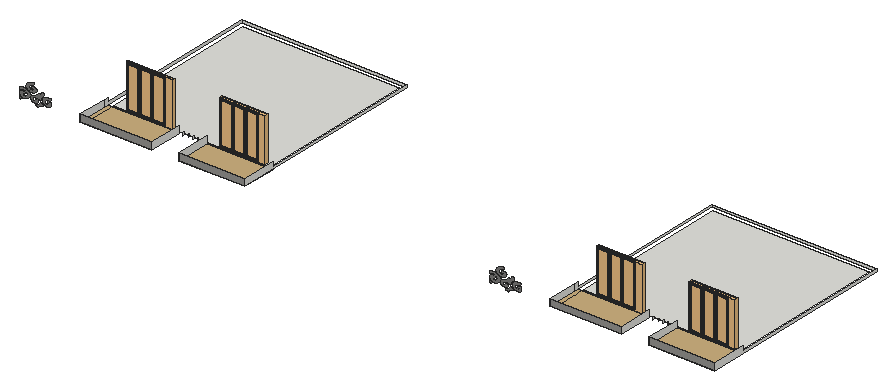
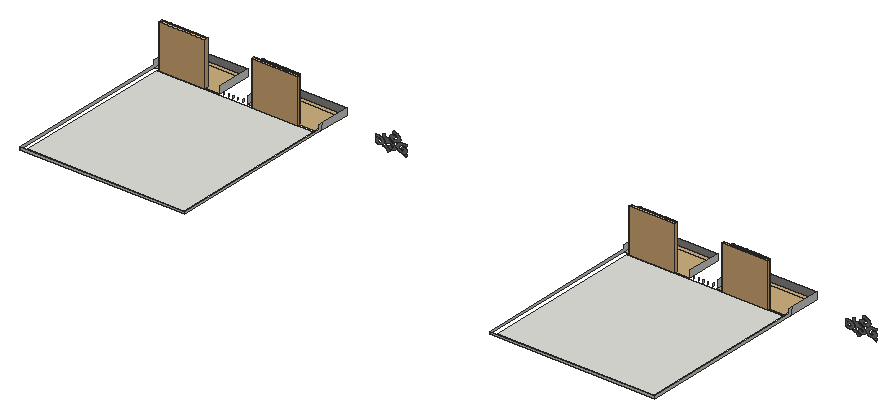
# SketchUp Ruby script. Lengths in inches.
U = 1.inch
M = Sketchup.active_model
def pt(a) = Geom::Point3d.new(a.map { |v| v * U })
def face(e, loops, mat)
  f = e.add_face(loops[0].map { |a| pt(a) })
  loops[1..].each { |l| e.add_face(l.map { |a| pt(a) }).erase! }
  f.material = f.back_material = mat if mat
  f
end
# faces: each face lists its corners as indices into pts; further lists are holes
def faces(e, pts, list, mat = nil) = list.each { |f| face(e, (f[0].is_a?(Array) ? f : [f]).map { |l| l.map { |i| pts[i] } }, mat) }
# xy, xz, yz: faces in a plane at the given z, y or x. An outline is a flat list of corners, or four numbers for a rectangle; further outlines are holes
def ring(l) = l.size == 4 ? [[l[0], l[1]], [l[2], l[1]], [l[2], l[3]], [l[0], l[3]]] : l.each_slice(2).to_a
def flat(e, list, mat, &to3) = list.each { |f| face(e, (f[0].is_a?(Array) ? f : [f]).map { |l| ring(l).map { |u, v| to3.(u, v) } }, mat) }
def xy(e, z, list, mat = nil) = flat(e, list, mat) { |x, y| [x, y, z] }
def xz(e, y, list, mat = nil) = flat(e, list, mat) { |x, z| [x, y, z] }
def yz(e, x, list, mat = nil) = flat(e, list, mat) { |y, z| [x, y, z] }
def lines(e, pts, list) = list.each { |a, b| e.add_line(pt(pts[a]), pt(pts[b])) }
# prism: a flat outline (further loops are holes) pulled along v
def prism(e, loops, v, mat = nil)
  f = face(e, loops, mat); d = Geom::Vector3d.new(v.map { |x| x * U })
  f.pushpull(f.normal.samedirection?(d) ? d.length : -d.length)
end
def box(e, o, s, mat = nil) = prism(e, [[o, [o[0] + s[0], o[1], o[2]], [o[0] + s[0], o[1] + s[1], o[2]], [o[0], o[1] + s[1], o[2]]]], [0, 0, s[2]], mat)
def at(x, y, z, deg = 0) = Geom::Transformation.translation(pt([x, y, z])) * Geom::Transformation.rotation(ORIGIN, Z_AXIS, deg.degrees)
def axes(o, x, y, z) = Geom::Transformation.new([*x, 0, *y, 0, *z, 0, *pt(o).to_a, 1])
def part(name) = M.definitions.add(name)
# library, detail: a bought-in or finely detailed component or shape, given as its bounding box
def library(name, o, s) = part(name).tap { |d| box(d.entities, o, s) }
def detail(e, o, s) = box(e.add_group.entities, o, s)
def put(e, d, t, mat = nil) = e.add_instance(d, t).tap { |i| i.material = mat if mat }
def group(e, t, mat = nil) = e.add_group.tap { |g| g.transformation = t; g.material = mat if mat }.entities
root = M.entities
M.materials.add("Wine2").color = [0, 0, 0]
M.materials["Wine2"].alpha = 0
M.materials.add("[0043_SaddleBrown]4").color = [124, 123, 122]
M.materials.add("[0130_Gainsboro]").color = [39, 45, 50]
M.materials.add("[Granite Light Gray]").color = [149, 148, 144]
M.materials.add("[Wood Floor Light]").color = [204, 176, 127]
c1 = part("Framed glazing panel")
xy(c1.entities,0,[[0,-0.98,43.07,0],[0,0,43.07,1.4]],"[0130_Gainsboro]")
xy(c1.entities,0.3,[[0.3,-1.43,42.77,-0.98]],"[0130_Gainsboro]")
xy(c1.entities,2.95,[[2.95,-1.43,40.12,-0.63],[2.95,-0.63,40.12,0],[2.95,0,40.12,0.64],[2.95,0.64,40.12,1.4]],"[0130_Gainsboro]")
xy(c1.entities,3.54,[[3.54,-0.63,39.53,0],[3.54,0,39.53,0.64]],"[0130_Gainsboro]")
xy(c1.entities,111.8125,[[3.54,-0.63,39.53,0],[3.54,0,39.53,0.64]],"[0130_Gainsboro]")
xy(c1.entities,112.4,[[2.95,-1.43,40.12,-0.63],[2.95,-0.63,40.12,0],[2.95,0,40.12,0.64],[2.95,0.64,40.12,1.4]],"[0130_Gainsboro]")
xy(c1.entities,115.05,[[0.3,-1.43,42.77,-0.98]],"[0130_Gainsboro]")
xy(c1.entities,115.35,[[0,-0.98,43.07,0],[0,0,43.07,1.4]],"[0130_Gainsboro]")
xz(c1.entities,-1.43,[[[0.3,0.3,42.77,115.05],[2.95,2.95,40.12,112.4]]],"[0130_Gainsboro]")
xz(c1.entities,-0.98,[[[0,0,43.07,115.35],[0.3,0.3,42.77,115.05]]],"[0130_Gainsboro]")
xz(c1.entities,-0.63,[[[2.95,2.95,40.12,112.4],[3.54,3.54,39.53,111.8125]]],"[0130_Gainsboro]")
xz(c1.entities,0,[[3.54,3.54,39.53,111.8125]],"Wine2")
xz(c1.entities,0,[[[0,0,43.07,115.35],[2.95,2.95,40.12,112.4]],[[2.95,2.95,40.12,112.4],[3.54,3.54,39.53,111.8125]]],"[0130_Gainsboro]")
xz(c1.entities,0.64,[[[2.95,2.95,40.12,112.4],[3.54,3.54,39.53,111.8125]]],"[0130_Gainsboro]")
xz(c1.entities,1.4,[[[0,0,43.07,115.35],[2.95,2.95,40.12,112.4]]],"[0130_Gainsboro]")
yz(c1.entities,0,[[-0.98,0,0,115.35],[0,0,1.4,115.35]],"[0130_Gainsboro]")
yz(c1.entities,0.3,[[-1.43,0.3,-0.98,115.05]],"[0130_Gainsboro]")
yz(c1.entities,2.95,[[-1.43,2.95,-0.63,112.4],[-0.63,2.95,0,112.4],[0,2.95,0.64,112.4],[0.64,2.95,1.4,112.4]],"[0130_Gainsboro]")
yz(c1.entities,3.54,[[-0.63,3.54,0,111.8125],[0,3.54,0.64,111.8125]],"[0130_Gainsboro]")
yz(c1.entities,39.53,[[-0.63,3.54,0,111.8125],[0,3.54,0.64,111.8125]],"[0130_Gainsboro]")
yz(c1.entities,40.12,[[-1.43,2.95,-0.63,112.4],[-0.63,2.95,0,112.4],[0,2.95,0.64,112.4],[0.64,2.95,1.4,112.4]],"[0130_Gainsboro]")
yz(c1.entities,42.77,[[-1.43,0.3,-0.98,115.05]],"[0130_Gainsboro]")
yz(c1.entities,43.07,[[-0.98,0,0,115.35],[0,0,1.4,115.35]],"[0130_Gainsboro]")
c2 = part("Glazing assembly")
put(c2.entities,c1,axes([90.57,1.43,0],[1.05148,0,0],[0,1,0],[0,0,1]))
put(c2.entities,c1,axes([0,1.43,0],[1.05148,0,0],[0,1,0],[0,0,1]))
put(c2.entities,c1,axes([45.29,1.43,0],[1.05148,0,0],[0,1,0],[0,0,1]))
c3 = library("Curtains",[0,0,0],[121.73,8.19,117.22])
xy(root,514.875,[[602.01,651.03,703.26,657.03],[849.76,651.03,951.01,657.03],[1852.64,651.03,1953.89,657.03],[2100.38,651.03,2201.63,657.03]])
xy(root,520.4375,[[563.08,657.03,978.86,1085.17],[1813.71,657.03,2229.49,1085.17]])
xy(root,520.4375,[[551.76,559.875,742.44,570.83],[814.89,559.875,990.19,570.83],[1802.38,559.875,1993.07,570.83],[2065.52,559.875,2240.81,570.83],[551.76,570.83,563.08,651.03],
  [563.08,570.83,742.44,651.03],[814.89,570.83,978.86,651.03],[978.86,570.83,990.19,651.03],[1802.38,570.83,1813.71,651.03],[1813.71,570.83,1993.07,651.03],
  [2065.52,570.83,2229.49,651.03],[2229.49,570.83,2240.81,651.03]],"[Wood Floor Light]")
xz(root,559.875,[[551.76,520.4375,742.44,538.1875],[814.89,520.4375,990.19,538.1875],[1802.38,520.4375,1993.07,538.1875],[2065.52,520.4375,2240.81,538.1875]],"[Granite Light Gray]")
xz(root,589.17,[[416.88,494.52,416.4,494.86,415.89,495.2,415.37,495.53,414.83,495.84,414.27,496.14,413.69,496.43,413.09,496.71,412.48,496.97,411.86,497.21,411.22,497.45,410.56,497.67,409.89,497.87,411.46,498.36,412.96,498.91,414.39,499.53,415.75,500.21,417.03,500.95,418.22,501.74,419.3125,502.59,420.3,503.48,421.19,504.4,421.97,505.37,422.63,506.37,423.18,507.39,423.73,507,424.29,506.61,424.86,506.23,425.44,505.86,426.04,505.49,426.64,505.13,427.25,504.77,427.87,504.42,429.13,503.74,429.78,503.41,430.4375,503.08,428.78,502.8125,427.17,502.44,425.625,501.98,424.16,501.42,422.8,500.78,421.54,500.0625,420.4,499.27,419.4,498.42,418.54,497.5,417.83,496.54,417.27,495.54],[1667.5,494.52,1667.02,494.86,1666.52,495.2,1666,495.53,1665.45,495.84,1664.89,496.14,1664.31,496.43,1663.72,496.71,1663.11,496.97,1662.48,497.21,1661.84,497.45,1661.19,497.67,1660.52,497.87,1662.08,498.36,1663.58,498.91,1665.02,499.53,1666.38,500.21,1667.66,500.95,1668.84,501.74,1669.9375,502.59,1670.93,503.48,1671.82,504.4,1672.59,505.37,1673.26,506.37,1673.8,507.39,1674.35,507,1674.92,506.61,1675.49,506.23,1676.07,505.86,1676.66,505.49,1677.26,505.13,1677.87,504.77,1678.49,504.42,1679.12,504.08,1679.76,503.74,1680.41,503.41,1681.0625,503.08,1679.4,502.8125,1677.79,502.44,1676.25,501.98,1674.79,501.42,1673.42,500.78,1672.16,500.0625,1671.03,499.27,1670.03,498.42,1669.16,497.5,1668.45,496.54,1667.9,495.54],[368.68,499.68,368.68,504.25,369.1,503.96,369.54,503.69,369.99,503.43,370.46,503.18,370.96,502.95,371.46,502.73,371.99,502.52,372.52,502.32,373.64,501.98,374.21,501.83,374.8,501.7,374.42,501.42,374.01,501.16,373.57,500.91,373.1,500.68,372.61,500.48,372.09,500.29,371.56,500.13,371.01,499.99,370.4375,499.875,369.86,499.78,369.28,499.72],[1619.31,499.68,1619.31,504.25,1619.72,503.96,1620.16,503.69,1620.62,503.43,1621.09,503.18,1621.58,502.95,1622.09,502.73,1622.61,502.52,1623.15,502.32,1623.7,502.15,1624.26,501.98,1624.84,501.83,1625.42,501.7,1625.04,501.42,1624.63,501.16,1624.19,500.91,1623.72,500.68,1623.23,500.48,1622.72,500.29,1622.18,500.13,1621.63,499.99,1621.0625,499.875,1620.49,499.78,1619.9,499.72],[406.11,502.53,404.67,502.63,403.28,502.875,401.97,503.24,400.76,503.73,399.6875,504.32,398.77,505.01,398.04,505.77,397.5,506.59,397.17,507.46,397.0625,508.34,396.95,509.36,397.01,510.38,397.25,511.39,397.65,512.39,398.22,513.35,398.95,514.27,399.83,515.14,400.85,515.94,402,516.68,403.27,517.34,404.64,517.92,406.1,518.41,407.49,518.85,408.83,519.35,410.1,519.91,411.3,520.53,412.43,521.19,413.49,521.91,414.45,522.66,415.33,523.46,416.11,524.29,416.79,525.16,417.38,526.05,417.86,526.96,418.53,526.65,419.27,526.39,420.07,526.2,420.89,526.08,421.74,526.02,422.59,526.04,423.42,526.13,424.24,526.28,425,526.51,425.72,526.79,426.36,527.13,426.92,527.52,427.13,527.84,427.28,528.17,427.36,528.51,427.38,528.85,427.34,529.18,427.24,529.52,427.08,529.85,426.86,530.16,426.58,530.45,426.25,530.73,425.875,530.98,425.45,531.2,425.22,531.33,425.04,531.48,424.91,531.66,424.84,531.85,424.83,532.04,424.875,532.23,424.98,532.41,425.15,532.57,425.36,532.71,425.61,532.83,425.9,532.91,426.2,532.95,426.76,532.98,427.32,532.95,427.86,532.875,428.38,532.75,428.87,532.59,429.32,532.38,429.71,532.14,430.04,531.86,430.31,531.56,430.5,531.24,430.61,530.9,430.65,530.56,430.86,529.99,431.01,529.41,431.09,528.83,431.09,528.24,431.03,527.66,430.9,527.08,430.7,526.5,430.43,525.94,430.1,525.39,429.7,524.86,429.24,524.35,428.72,523.86,427.79,523,426.92,522.11,426.11,521.2,425.375,520.27,424.71,519.33,424.11,518.36,423.59,517.375,423.14,516.38,422.76,515.375,422.46,514.36,422.23,513.33,422.08,512.3,421.11,513.07,419.99,513.75,418.74,514.33,417.37,514.8125,415.91,515.18,414.39,515.42,412.83,515.55,411.25,515.54,409.6875,515.42,408.17,515.16,406.71,514.79,405.35,514.31,404.375,513.85,403.51,513.32,402.76,512.72,402.14,512.07,401.66,511.38,401.33,510.65,401.16,509.91,401.14,509.15,401.28,508.41,401.58,507.67,402.03,506.97,402.62,506.3125,403.16,506.0625,403.76,505.86,404.41,505.72,405.08,505.64,405.76,505.62,406.4375,505.66,407.1,505.77,407.73,505.93,408.31,506.16,408.83,506.43,409.28,506.74,409.64,507.1,409.52,507.35,409.4375,507.61,409.38,507.87,409.36,508.125,409.38,508.39,409.43,508.65,409.51,508.91,409.62,509.16,409.77,509.4,409.94,509.64,410.15,509.87,410.39,510.09,410.62,510.26,410.89,510.4,411.2,510.51,411.53,510.6,411.88,510.65,412.24,510.67,412.59,510.65,412.94,510.6,413.27,510.51,413.58,510.4,413.85,510.26,414.08,510.09,414.76,509.4,415.23,508.65,415.49,507.87,415.52,507.07,415.33,506.27,414.92,505.51,414.3125,504.8,413.51,504.17,412.55,503.63,411.45,503.2,410.24,502.89,408.97,502.71,407.55,502.55],
  [1656.73,502.53,1655.3,502.63,1653.91,502.875,1652.59,503.24,1651.39,503.73,1650.3125,504.32,1649.4,505.01,1648.66,505.77,1648.125,506.59,1647.8,507.46,1647.6875,508.34,1647.58,509.36,1647.64,510.38,1647.87,511.39,1648.28,512.39,1648.84,513.35,1649.57,514.27,1650.45,515.14,1651.47,515.94,1652.62,516.68,1653.89,517.34,1655.27,517.92,1656.73,518.41,1658.12,518.85,1659.45,519.35,1660.72,519.91,1661.93,520.53,1663.06,521.19,1664.11,521.91,1665.08,522.66,1665.95,523.46,1666.74,524.29,1667.42,525.16,1668,526.05,1668.48,526.96,1669.16,526.65,1669.9,526.39,1670.69,526.2,1671.52,526.08,1672.36,526.02,1673.21,526.04,1674.05,526.13,1674.86,526.28,1675.63,526.51,1676.34,526.79,1676.99,527.13,1677.55,527.52,1677.75,527.84,1677.9,528.17,1677.99,528.51,1678.01,528.85,1677.97,529.18,1677.87,529.52,1677.7,529.85,1677.48,530.16,1677.21,530.45,1676.875,530.73,1676.5,530.98,1676.08,531.2,1675.85,531.33,1675.66,531.48,1675.53,531.66,1675.46,531.85,1675.45,532.04,1675.5,532.23,1675.61,532.41,1675.77,532.57,1675.99,532.71,1676.24,532.83,1676.52,532.91,1676.83,532.95,1677.38,532.98,1677.94,532.95,1678.49,532.875,1679.01,532.75,1679.5,532.59,1679.94,532.38,1680.33,532.14,1680.67,531.86,1680.93,531.56,1681.12,531.24,1681.24,530.9,1681.27,530.56,1681.49,529.99,1681.63,529.41,1681.71,528.83,1681.72,528.24,1681.66,527.66,1681.52,527.08,1681.32,526.5,1681.06,525.94,1680.72,525.39,1680.33,524.86,1679.87,524.35,1679.35,523.86,1678.41,523,1677.54,522.11,1676.74,521.2,1676,520.27,1675.33,519.33,1674.74,518.36,1674.21,517.375,1673.76,516.38,1673.38,515.375,1673.08,514.36,1672.86,513.33,1672.7,512.3,1671.74,513.07,1670.62,513.75,1669.36,514.33,1667.99,514.8125,1666.54,515.18,1665.01,515.42,1663.45,515.55,1661.875,515.54,1660.3125,515.42,1658.79,515.16,1657.34,514.79,1655.97,514.31,1655,513.85,1654.13,513.32,1653.38,512.72,1652.76,512.07,1652.29,511.38,1651.96,510.65,1651.78,509.91,1651.77,509.15,1651.91,508.41,1652.2,507.67,1652.65,506.97,1653.24,506.3125,1653.79,506.0625,1654.39,505.86,1655.03,505.72,1655.7,505.64,1656.38,505.62,1657.0625,505.66,1657.72,505.77,1658.35,505.93,1658.93,506.16,1659.45,506.43,1659.9,506.74,1660.27,507.1,1660.15,507.35,1660.0625,507.61,1660.01,507.87,1659.99,508.125,1660,508.39,1660.05,508.65,1660.13,508.91,1660.25,509.16,1660.39,509.4,1660.57,509.64,1660.78,509.87,1661.01,510.09,1661.25,510.26,1661.52,510.4,1661.82,510.51,1662.16,510.6,1662.5,510.65,1662.86,510.67,1663.22,510.65,1663.57,510.6,1663.9,510.51,1664.2,510.4,1664.48,510.26,1664.71,510.09,1665.38,509.4,1665.85,508.65,1666.11,507.87,1666.15,507.07,1665.96,506.27,1665.55,505.51,1664.9375,504.8,1664.14,504.17,1663.17,503.63,1662.07,503.2,1660.87,502.89,1659.59,502.71,1658.17,502.55],[378.83,503.5,377.68,503.64,376.54,503.84,375.45,504.11,374.4,504.44,373.4,504.83,372.47,505.28,371.62,505.78,370.84,506.32,370.15,506.91,369.5625,507.54,369.07,508.2,368.68,508.88,368.68,515.77,369.21,516.54,369.99,517.23,370.98,517.81,372.13,518.25,373.41,518.54,374.76,518.66,376.12,518.61,377.4375,518.39,378.66,518.01,379.72,517.49,380.59,516.85,381.23,516.11,381.32,515.93,381.375,515.75,381.38,515.56,381.34,515.375,381.26,515.19,381.13,515.02,380.97,514.87,380.76,514.72,380.53,514.6,380.27,514.51,379.99,514.43,379.7,514.38,378.97,514.46,378.24,514.45,377.51,514.36,376.83,514.19,376.21,513.95,375.67,513.64,375.24,513.27,374.92,512.86,374.74,512.42,374.68,511.97,374.76,511.52,374.98,511.09,375.16,510.53,375.49,509.99,375.94,509.49,376.52,509.04,377.21,508.65,377.99,508.34,378.84,508.1,379.74,507.95,380.67,507.89,381.6,507.91,382.51,508.03,383.39,508.24,384.74,508.91,385.93,509.6875,386.93,510.5625,387.71,511.52,388.27,512.53,388.59,513.58,388.66,514.65,388.49,515.71,388.07,516.75,387.42,517.74,386.54,518.67,385.47,519.51,385.03,520.06,384.51,520.6,383.93,521.1,383.28,521.57,382.57,522.01,381.81,522.41,380.99,522.77,380.12,523.08,379.22,523.35,378.28,523.58,377.32,523.75,376.33,523.875,375.63,523.93,374.92,523.94,374.22,523.92,373.52,523.86,372.83,523.77,372.15,523.64,371.5,523.48,370.87,523.28,370.27,523.05,369.7,522.8,369.17,522.51,368.68,522.2,368.68,526.94,370.83,527.38,373.04,527.66,375.3,527.78,377.56,527.72,379.79,527.51,381.97,527.125,384.05,526.59,386.02,525.9,387.84,525.07,389.48,524.12,390.93,523.05,392.16,521.88,393.82,520.15,394.98,518.26,395.59,516.28,395.64,514.26,395.12,512.26,394.05,510.36,392.45,508.59,390.39,507.02,387.92,505.69,385.11,504.64,382.05,503.91],[1629.46,503.5,1628.3,503.64,1627.17,503.84,1626.07,504.11,1625.02,504.44,1624.03,504.83,1623.1,505.28,1622.24,505.78,1621.47,506.32,1620.78,506.91,1620.1875,507.54,1619.7,508.2,1619.31,508.88,1619.31,515.77,1619.84,516.54,1620.61,517.23,1621.6,517.81,1622.76,518.25,1624.04,518.54,1625.39,518.66,1626.75,518.61,1628.0625,518.39,1629.28,518.01,1630.35,517.49,1631.22,516.85,1631.86,516.11,1631.95,515.93,1632,515.75,1632,515.56,1631.97,515.375,1631.88,515.19,1631.76,515.02,1631.59,514.87,1631.39,514.72,1631.16,514.6,1630.9,514.51,1630.62,514.43,1630.32,514.38,1629.6,514.46,1628.86,514.45,1628.14,514.36,1627.46,514.19,1626.84,513.95,1626.3,513.64,1625.87,513.27,1625.55,512.86,1625.36,512.42,1625.31,511.97,1625.39,511.52,1625.6,511.09,1625.79,510.53,1626.11,509.99,1626.57,509.49,1627.15,509.04,1627.84,508.65,1628.62,508.34,1629.47,508.1,1630.37,507.95,1631.29,507.89,1632.23,507.91,1633.14,508.03,1634.01,508.24,1635.37,508.91,1636.56,509.6875,1637.55,510.5625,1638.34,511.52,1638.89,512.53,1639.21,513.58,1639.28,514.65,1639.11,515.71,1638.69,516.75,1638.04,517.74,1637.17,518.67,1636.09,519.51,1635.65,520.06,1635.14,520.6,1634.56,521.1,1633.91,521.57,1633.2,522.01,1632.43,522.41,1631.61,522.77,1630.75,523.08,1629.84,523.35,1628.91,523.58,1627.94,523.75,1626.96,523.875,1626.25,523.93,1625.55,523.94,1624.84,523.92,1624.14,523.86,1623.45,523.77,1622.78,523.64,1622.125,523.48,1621.49,523.28,1620.89,523.05,1620.33,522.8,1619.8,522.51,1619.31,522.2,1619.31,526.94,1621.45,527.38,1623.67,527.66,1625.92,527.78,1628.18,527.72,1630.42,527.51,1632.59,527.125,1634.68,526.59,1636.64,525.9,1638.46,525.07,1640.11,524.12,1641.55,523.05,1642.78,521.88,1644.45,520.15,1645.61,518.26,1646.22,516.28,1646.26,514.26,1645.74,512.26,1644.67,510.36,1643.08,508.59,1641.02,507.02,1638.55,505.69,1635.74,504.64,1632.68,503.91],[441.63,504.03,440.28,504.08,438.94,504.23,437.65,504.49,436.41,504.83,435.25,505.27,434.19,505.79,433.3,506.32,432.47,506.89,431.69,507.49,430.99,508.12,430.36,508.78,429.8,509.46,429.32,510.16,428.91,510.89,428.58,511.625,428.34,512.37,428.18,513.13,428.1,513.89,428.21,515.5,428.72,517.08,429.61,518.59,430.86,520.01,432.44,521.29,434.32,522.41,436.45,523.35,438.79,524.07,441.27,524.58,443.86,524.85,446.48,524.875,449.07,524.66,449.07,520.65,446.84,520.7,444.63,520.51,442.51,520.08,440.54,519.43,438.79,518.59,437.3,517.57,436.12,516.41,435.29,515.13,434.83,513.79,434.76,512.42,435.07,511.07,435.77,509.76,436.5625,509.21,437.52,508.75,438.59,508.42,439.75,508.21,440.95,508.14,442.15,508.21,443.31,508.42,444.38,508.76,445.33,509.22,446.125,509.78,446.73,510.42,447.13,511.12,447.21,511.4,447.2,511.6875,447.11,511.97,446.95,512.24,446.71,512.49,446.41,512.71,446.05,512.89,445.65,513.03,445.21,513.13,444.75,513.1875,444.28,513.1875,443.82,513.14,443.57,513.21,443.35,513.29,443.13,513.39,442.9375,513.5,442.76,513.62,442.61,513.75,442.48,513.89,442.38,514.04,442.3,514.2,442.26,514.36,442.24,514.52,442.24,514.68,442.61,515.01,443.05,515.31,443.55,515.57,444.1,515.78,444.6875,515.95,445.31,516.07,445.95,516.14,446.6,516.16,447.25,516.12,447.89,516.03,448.5,515.89,449.07,515.7,449.07,505.79,448.01,505.27,446.86,504.83,445.62,504.49,444.32,504.23,442.99,504.08],[1692.26,504.03,1690.9,504.08,1689.57,504.23,1688.27,504.49,1687.04,504.83,1685.88,505.27,1684.82,505.79,1683.92,506.32,1683.09,506.89,1682.32,507.49,1681.62,508.12,1680.98,508.78,1680.42,509.46,1679.94,510.16,1679.54,510.89,1679.21,511.625,1678.96,512.37,1678.8,513.13,1678.72,513.89,1678.84,515.5,1679.35,517.08,1680.24,518.59,1681.49,520.01,1683.07,521.29,1684.94,522.41,1687.08,523.35,1689.41,524.07,1691.9,524.58,1694.48,524.85,1697.1,524.875,1699.7,524.66,1699.7,520.65,1697.47,520.7,1695.26,520.51,1693.14,520.08,1691.17,519.43,1689.41,518.59,1687.92,517.57,1686.75,516.41,1685.91,515.13,1685.45,513.79,1685.38,512.42,1685.7,511.07,1686.39,509.76,1687.1875,509.21,1688.14,508.75,1689.22,508.42,1690.375,508.21,1691.58,508.14,1692.78,508.21,1693.94,508.42,1695.01,508.76,1695.96,509.22,1696.75,509.78,1697.36,510.42,1697.76,511.12,1697.83,511.4,1697.82,511.6875,1697.74,511.97,1697.57,512.24,1697.34,512.49,1697.03,512.71,1696.68,512.89,1696.27,513.03,1695.83,513.13,1695.37,513.1875,1694.9,513.1875,1694.44,513.14,1694.2,513.21,1693.97,513.29,1693.76,513.39,1693.5625,513.5,1693.39,513.62,1693.24,513.75,1693.11,513.89,1693.01,514.04,1692.93,514.2,1692.88,514.36,1692.86,514.52,1692.87,514.68,1693.24,515.01,1693.67,515.31,1694.17,515.57,1694.72,515.78,1695.3125,515.95,1695.93,516.07,1696.57,516.14,1697.23,516.16,1697.875,516.12,1698.51,516.03,1699.12,515.89,1699.7,515.7,1699.7,505.79,1698.64,505.27,1697.48,504.83,1696.24,504.49,1694.95,504.23,1693.61,504.08],
  [399.52,524.15,397.1875,524.23,394.9,524.54,392.72,525.06,390.7,525.78,388.89,526.69,387.34,527.76,386.07,528.97,385.125,530.28,384.52,531.67,384.29,533.1,384.41,534.54,384.9,535.94,385.46,537.31,386.21,538.63,387.17,539.91,388.31,541.13,389.62,542.28,391.1,543.35,392.74,544.33,394.52,545.22,396.42,546,398.43,546.68,400.53,547.23,402.71,547.67,403.12,547.29,403.48,546.89,403.8,546.47,404.06,546.05,404.27,545.61,404.42,545.16,404.53,544.71,404.57,544.26,404.56,543.8,404.49,543.35,404.375,542.9,404.2,542.45,402.85,542.55,401.49,542.53,400.14,542.4,398.84,542.15,397.61,541.8,396.47,541.34,395.4375,540.79,394.54,540.17,393.8,539.47,393.21,538.71,392.81,537.91,392.58,537.09,392.22,536.31,391.99,535.51,391.9,534.7,391.95,533.89,392.14,533.09,392.47,532.31,392.94,531.55,393.54,530.82,394.25,530.14,395.09,529.51,396.03,528.94,397.06,528.4375,398.01,528.1,399.06,527.875,400.15,527.78,401.26,527.81,402.33,527.97,403.34,528.25,404.24,528.64,405.01,529.13,405.61,529.7,406.02,530.33,406.24,531,406.24,531.68,406.15,532.01,405.99,532.34,405.76,532.64,405.47,532.93,405.11,533.1875,404.7,533.41,404.24,533.6,403.74,533.75,403.22,533.86,402.68,533.92,402.125,533.9375,401.58,533.91,401,533.89,400.4375,533.96,399.91,534.1,399.45,534.3125,399.09,534.58,398.83,534.9,398.69,535.24,398.6875,535.59,398.8125,535.9375,399.0625,536.25,399.42,536.53,399.875,536.75,401.12,537.12,402.46,537.35,403.84,537.43,405.23,537.35,406.5625,537.125,407.81,536.75,408.93,536.24,409.87,535.61,410.62,534.89,411.14,534.1,411.42,533.27,411.44,532.41,411.5,531.38,411.32,530.35,410.92,529.35,410.29,528.39,409.46,527.49,408.43,526.68,407.23,525.95,405.88,525.33,404.41,524.84,402.84,524.47,401.2,524.24],[1650.15,524.15,1647.8125,524.23,1645.53,524.54,1643.35,525.06,1641.33,525.78,1639.52,526.69,1637.96,527.76,1636.69,528.97,1635.75,530.28,1635.15,531.67,1634.91,533.1,1635.04,534.54,1635.53,535.94,1636.08,537.31,1636.84,538.63,1637.79,539.91,1638.93,541.13,1640.25,542.28,1641.73,543.35,1643.37,544.33,1645.14,545.22,1647.04,546,1649.05,546.68,1651.16,547.23,1653.33,547.67,1653.74,547.29,1654.11,546.89,1654.42,546.47,1654.68,546.05,1654.89,545.61,1655.05,545.16,1655.15,544.71,1655.2,544.26,1655.19,543.8,1655.12,543.35,1655,542.9,1654.82,542.45,1653.47,542.55,1652.11,542.53,1650.77,542.4,1649.47,542.15,1648.23,541.8,1647.09,541.34,1646.0625,540.79,1645.17,540.17,1644.42,539.47,1643.84,538.71,1643.43,537.91,1643.21,537.09,1642.84,536.31,1642.61,535.51,1642.52,534.7,1642.57,533.89,1642.77,533.09,1643.1,532.31,1643.56,531.55,1644.16,530.82,1644.88,530.14,1645.71,529.51,1646.65,528.94,1647.68,528.4375,1648.64,528.1,1649.68,527.875,1650.78,527.78,1651.88,527.81,1652.96,527.97,1653.97,528.25,1654.87,528.64,1655.63,529.13,1656.24,529.7,1656.65,530.33,1656.86,531,1656.87,531.68,1656.78,532.01,1656.62,532.34,1656.39,532.64,1656.09,532.93,1655.73,533.1875,1655.32,533.41,1654.86,533.6,1654.37,533.75,1653.85,533.86,1653.3,533.92,1652.75,533.9375,1652.2,533.91,1651.63,533.89,1651.0625,533.96,1650.54,534.1,1650.08,534.3125,1649.71,534.58,1649.45,534.9,1649.32,535.24,1649.3125,535.59,1649.4375,535.9375,1649.6875,536.25,1650.05,536.53,1650.5,536.75,1651.75,537.12,1653.08,537.35,1654.47,537.43,1655.85,537.35,1657.1875,537.125,1658.44,536.75,1659.55,536.24,1660.5,535.61,1661.24,534.89,1661.76,534.1,1662.04,533.27,1662.07,532.41,1662.12,531.38,1661.95,530.35,1661.54,529.35,1660.92,528.39,1660.08,527.49,1659.06,526.68,1657.86,525.95,1656.51,525.33,1655.03,524.84,1653.46,524.47,1651.82,524.24]],"[0043_SaddleBrown]4")
xz(root,1096.5,[[551.76,520.4375,990.19,526.4375],[1802.38,520.4375,2240.81,526.4375]])
yz(root,551.76,[[559.875,520.4375,640.11,538.1875],[640.11,520.4375,640.11,538.1875,651.03,538.1875,651.03,526.4375,1096.5,526.4375,1096.5,520.4375]])
yz(root,742.44,[[559.875,520.4375,647.91,538.1875]])
yz(root,755.44,[[647.91,520.4375,651.03,526.4375]])
yz(root,768.19,[[648.85,520.4375,651.03,526.4375]])
yz(root,780.32,[[648.85,520.4375,651.03,526.4375]])
yz(root,792.69,[[648.85,520.4375,651.03,526.4375]])
yz(root,805.57,[[648.85,520.4375,651.03,526.4375]])
yz(root,814.89,[[559.875,520.4375,651.03,538.1875]])
yz(root,990.19,[[559.875,520.4375,1096.5,520.4375,1096.5,526.4375,651.03,526.4375,651.03,538.1875,559.875,538.1875]])
yz(root,1802.38,[[559.875,520.4375,640.11,538.1875],[640.11,520.4375,640.11,538.1875,651.03,538.1875,651.03,526.4375,1096.5,526.4375,1096.5,520.4375]])
yz(root,1993.07,[[559.875,520.4375,647.91,538.1875]])
yz(root,2006.07,[[647.91,520.4375,651.03,526.4375]])
yz(root,2018.82,[[648.85,520.4375,651.03,526.4375]])
yz(root,2030.94,[[648.85,520.4375,651.03,526.4375]])
yz(root,2043.32,[[648.85,520.4375,651.03,526.4375]])
yz(root,2056.19,[[648.85,520.4375,651.03,526.4375]])
yz(root,2065.52,[[559.875,520.4375,651.03,538.1875]])
yz(root,2240.81,[[559.875,520.4375,1096.5,520.4375,1096.5,526.4375,651.03,526.4375,651.03,538.1875,559.875,538.1875]])
p = [[368.68,589.17,496.56],[368.68,589.17,499.68],[1619.31,589.17,496.56],[1619.31,589.17,499.68]]
lines(root,p,[[0,1],[2,3]])
put(root,c2,axes([601.61,650.7,523.79],[0.75,0,0],[0,0.75,0],[0,0,1.01765]))
put(root,c3,at(602.04,651.77,521.91))
put(root,c2,axes([849.11,651.03,523.48],[0.75,0,0],[0,0.75,0],[0,0,1.01765]))
put(root,c3,at(847.86,652.22,523.95))
put(root,c2,axes([1852.23,650.7,523.79],[0.75,0,0],[0,0.75,0],[0,0,1.01765]))
put(root,c3,at(1852.66,651.77,521.91))
put(root,c2,axes([2099.73,651.03,523.48],[0.75,0,0],[0,0.75,0],[0,0,1.01765]))
put(root,c3,at(2098.49,652.22,523.95))
